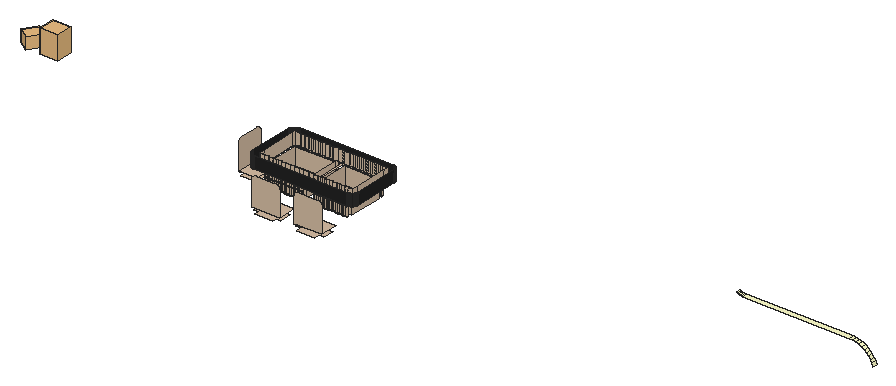
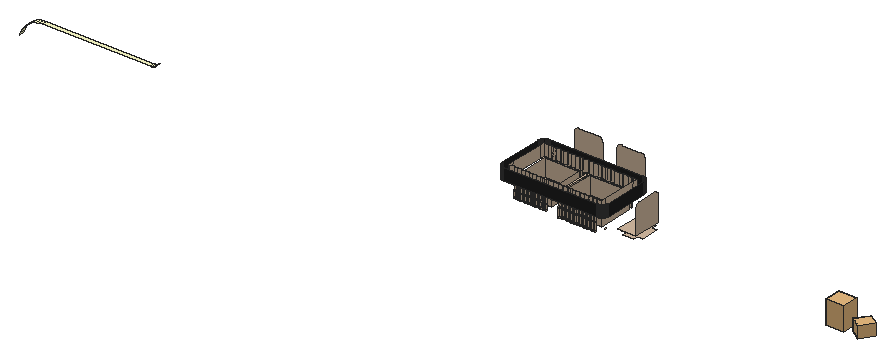
# SketchUp Ruby script. Lengths in inches.
U = 1.inch
M = Sketchup.active_model
def pt(a) = Geom::Point3d.new(a.map { |v| v * U })
def face(e, loops, mat)
  f = e.add_face(loops[0].map { |a| pt(a) })
  loops[1..].each { |l| e.add_face(l.map { |a| pt(a) }).erase! }
  f.material = f.back_material = mat if mat
  f
end
# faces: each face lists its corners as indices into pts; further lists are holes
def faces(e, pts, list, mat = nil) = list.each { |f| face(e, (f[0].is_a?(Array) ? f : [f]).map { |l| l.map { |i| pts[i] } }, mat) }
# xy, xz, yz: faces in a plane at the given z, y or x. An outline is a flat list of corners, or four numbers for a rectangle; further outlines are holes
def ring(l) = l.size == 4 ? [[l[0], l[1]], [l[2], l[1]], [l[2], l[3]], [l[0], l[3]]] : l.each_slice(2).to_a
def flat(e, list, mat, &to3) = list.each { |f| face(e, (f[0].is_a?(Array) ? f : [f]).map { |l| ring(l).map { |u, v| to3.(u, v) } }, mat) }
def xy(e, z, list, mat = nil) = flat(e, list, mat) { |x, y| [x, y, z] }
def xz(e, y, list, mat = nil) = flat(e, list, mat) { |x, z| [x, y, z] }
def yz(e, x, list, mat = nil) = flat(e, list, mat) { |y, z| [x, y, z] }
def lines(e, pts, list) = list.each { |a, b| e.add_line(pt(pts[a]), pt(pts[b])) }
# prism: a flat outline (further loops are holes) pulled along v
def prism(e, loops, v, mat = nil)
  f = face(e, loops, mat); d = Geom::Vector3d.new(v.map { |x| x * U })
  f.pushpull(f.normal.samedirection?(d) ? d.length : -d.length)
end
def box(e, o, s, mat = nil) = prism(e, [[o, [o[0] + s[0], o[1], o[2]], [o[0] + s[0], o[1] + s[1], o[2]], [o[0], o[1] + s[1], o[2]]]], [0, 0, s[2]], mat)
def at(x, y, z, deg = 0) = Geom::Transformation.translation(pt([x, y, z])) * Geom::Transformation.rotation(ORIGIN, Z_AXIS, deg.degrees)
def axes(o, x, y, z) = Geom::Transformation.new([*x, 0, *y, 0, *z, 0, *pt(o).to_a, 1])
def part(name) = M.definitions.add(name)
# library, detail: a bought-in or finely detailed component or shape, given as its bounding box
def library(name, o, s) = part(name).tap { |d| box(d.entities, o, s) }
def detail(e, o, s) = box(e.add_group.entities, o, s)
def put(e, d, t, mat = nil) = e.add_instance(d, t).tap { |i| i.material = mat if mat }
def group(e, t, mat = nil) = e.add_group.tap { |g| g.transformation = t; g.material = mat if mat }.entities
root = M.entities
M.materials.add("[0136_Charcoal]").color = [35, 35, 35]
M.materials.add("[Color E01]").color = [255, 255, 204]
M.materials.add("[Formica Laminate Light]").color = [213, 189, 164]
c1 = library("Vase 004",[-7.23,-6.39,-0.02],[13.74,12.68,17.81])
c2 = library("Books 155 025",[-5.0625,-5.83,0.01],[10.11,11.66,8.59])
xy(root,25.5625,[[268.91,97.95,268.91,101.59,265.27,101.59,265.27,110.07,268.72,110.07,268.72,113.72,282.83,113.72,282.83,110.07,286.47,110.07,286.47,101.59,282.83,101.59,282.83,97.95],[301.53,97.95,301.53,101.59,297.89,101.59,297.89,110.07,301.35,110.07,301.35,113.72,315.45,113.72,315.45,110.07,319.1,110.07,319.1,101.59,315.45,101.59,315.45,97.95],[233.08,129.3,233.08,132.94,229.44,132.94,229.44,146.86,233.08,146.86,233.08,150.5,241.57,150.5,241.57,147.05,245.21,147.05,245.21,132.94,241.57,132.94,241.57,129.3]],"[Formica Laminate Light]")
xy(root,26.83,[[255.19,159.08,257.64,160.01],[258.46,159.08,260.91,160.01],[261.72,159.08,264.17,160.01],[264.98,159.08,267.43,160.01],[268.24,159.08,270.69,160.01],
  [271.5,159.08,273.95,160.01],[274.76,159.08,277.21,160.01],[278.02,159.08,280.47,160.01],[281.29,159.08,283.74,160.01]],"[Formica Laminate Light]")
xy(root,27.63,[[255.19,159.08,257.64,160.01],[258.46,159.08,260.91,160.01],[261.72,159.08,264.17,160.01],[268.24,159.08,270.69,160.01],[271.5,159.08,273.95,160.01],
  [274.76,159.08,277.21,160.01],[278.02,159.08,280.47,160.01],[281.29,159.08,283.74,160.01]],"[Formica Laminate Light]")
xy(root,27.64,[[264.98,159.08,267.43,160.01]],"[Formica Laminate Light]")
xy(root,27.9,[[293.16,159.08,295.2,159.77],[296.03,159.08,298.0625,159.77],[298.89,159.08,300.93,159.77],[301.75,159.08,303.79,159.77],[304.62,159.08,306.66,159.77],
  [307.48,159.08,309.52,159.77],[310.35,159.08,312.38,159.77],[313.21,159.08,315.25,159.77],[316.07,159.08,318.11,159.77]],"[Formica Laminate Light]")
xy(root,28.25,[[265.27,99.82,286.47,113.72],[297.89,99.82,319.1,113.72],[231.32,129.3,245.21,150.5]],"[Formica Laminate Light]")
xy(root,28.4,[[254.81,124.84,257.68,125.33],[258.11,124.84,260.98,125.33],[261.41,124.84,264.28,125.33],[264.71,124.84,267.58,125.33],[268.02,124.84,270.89,125.33],
  [271.32,124.84,274.19,125.33],[274.625,124.84,277.49,125.33],[277.93,124.84,280.8,125.33],[281.23,124.84,284.1,125.33]],"[Formica Laminate Light]")
xy(root,28.69,[[254.38,128.96,284.55,155.08],[292.34,128.96,318.9375,155.08],[250.94,155.08,250.9,155.58,250.93,156.07,250.94,156.11],[293.16,159.08,295.2,159.77],[296.03,159.08,298.0625,159.77],
  [298.89,159.08,300.93,159.77],[301.75,159.08,303.79,159.77],[304.62,159.08,306.66,159.77],[307.48,159.08,309.52,159.77],[310.35,159.08,312.38,159.77],
  [313.21,159.08,315.25,159.77],[316.07,159.08,318.11,159.77]],"[Formica Laminate Light]")
xy(root,28.96,[[292.63,124.79,295.1875,125.33],[295.55,124.79,298.11,125.33],[298.47,124.79,301.04,125.33],[301.4,124.79,303.96,125.33],[304.32,124.79,306.88,125.33],
  [307.24,124.79,309.81,125.33],[310.17,124.79,312.73,125.33],[313.09,124.79,315.65,125.33],[316.01,124.79,318.58,125.33]],"[Formica Laminate Light]")
xy(root,32.6875,[[293.16,159.08,295.2,159.77],[296.03,159.08,298.0625,159.77],[298.89,159.08,300.93,159.77],[301.75,159.08,303.79,159.77],[304.62,159.08,306.66,159.77],
  [307.48,159.08,309.52,159.77],[310.35,159.08,312.38,159.77],[313.21,159.08,315.25,159.77],[316.07,159.08,318.11,159.77]],"[Formica Laminate Light]")
xy(root,33.4,[[255.19,159.08,257.64,160.01],[258.46,159.08,260.91,160.01],[261.72,159.08,264.17,160.01],[264.98,159.08,267.43,160.01],[268.24,159.08,270.69,160.01],
  [271.5,159.08,273.95,160.01],[274.76,159.08,277.21,160.01],[278.02,159.08,280.47,160.01],[281.29,159.08,283.74,160.01]],"[Formica Laminate Light]")
xy(root,33.49,[[293.16,159.08,295.2,159.77],[296.03,159.08,298.0625,159.77],[298.89,159.08,300.93,159.77],[301.75,159.08,303.79,159.77],[304.62,159.08,306.66,159.77],
  [307.48,159.08,309.52,159.77],[310.35,159.08,312.38,159.77],[313.21,159.08,315.25,159.77],[316.07,159.08,318.11,159.77]],"[Formica Laminate Light]")
xy(root,34.17,[[254.81,124.84,257.68,125.33],[258.11,124.84,260.98,125.33],[261.41,124.84,264.28,125.33],[264.71,124.84,267.58,125.33],[268.02,124.84,270.89,125.33],
  [271.32,124.84,274.19,125.33],[274.625,124.84,277.49,125.33],[277.93,124.84,280.8,125.33],[281.23,124.84,284.1,125.33]],"[Formica Laminate Light]")
xy(root,34.2,[[255.19,159.08,257.64,160.01],[258.46,159.08,260.91,160.01],[268.24,159.08,270.69,160.01],[271.5,159.08,273.95,160.01],[274.76,159.08,277.21,160.01],
  [278.02,159.08,280.47,160.01],[281.29,159.08,283.74,160.01]],"[Formica Laminate Light]")
xy(root,34.21,[[261.72,159.08,264.17,160.01]],"[Formica Laminate Light]")
xy(root,34.22,[[264.98,159.08,267.43,160.01]],"[Formica Laminate Light]")
xy(root,36.25,[[292.63,124.91,295.1875,125.45],[295.55,124.91,298.11,125.45],[298.47,124.91,301.04,125.45],[301.4,124.91,303.96,125.45],[304.32,124.91,306.88,125.45],
  [307.24,124.91,309.81,125.45],[310.17,124.91,312.73,125.45],[313.09,124.91,315.65,125.45],[316.01,124.91,318.58,125.45]],"[Formica Laminate Light]")
xy(root,39.6875,[[577,182.5625,659.67,185.9375]],"[Color E01]")
xy(root,40.33,[[[251.07,119.96,250.37,120,249.68,120.14,249.01,120.37,248.38,120.68,247.8,121.07,247.27,121.53,246.81,122.06,246.42,122.64,246.11,123.27,245.88,123.9375,245.74,124.625,245.7,125.33,245.7,159.08,245.8,159.73,245.97,160.35,246.22,160.95,246.54,161.52,246.93,162.04,247.39,162.51,247.89,162.91,248.44,163.26,249.03,163.53,249.65,163.73,250.29,163.85,250.94,163.89,322.35,163.89,323,163.85,323.63,163.73,324.24,163.53,324.82,163.25,325.37,162.91,325.86,162.5,326.3,162.03,326.68,161.51,326.99,160.94,327.22,160.34,327.38,159.72,327.46,159.08,327.46,125.33,327.42,124.65,327.29,123.98,327.08,123.33,326.78,122.72,326.42,122.14,325.98,121.62,325.48,121.16,324.93,120.76,324.33,120.44,323.69,120.2,323.03,120.03,322.35,119.96],[318.58,124.79,318.9375,124.79,318.9375,125.33,322.35,125.33,322.35,159.08,318.9375,159.08,318.9375,159.77,318.11,159.77,318.11,159.08,284.55,159.08,284.55,160.01,283.74,160.01,283.74,159.08,250.94,159.08,250.94,125.33,284.1,125.33,284.1,124.84,284.53,124.84,284.53,125.33,318.58,125.33]],[250.94,125.33,250.94,128.96,251.03,128.53,251.16,128.11,251.34,127.7,251.55,127.3125,251.81,126.95,252.09,126.61,252.42,126.3,252.77,126.03,253.14,125.79,253.54,125.6,253.95,125.44,254.38,125.33],[284.53,125.33,284.96,125.41,285.38,125.55,285.78,125.73,286.16,125.96,286.5,126.23,286.8125,126.55,287.08,126.89,287.31,127.27,287.49,127.67,287.62,128.09,287.69,128.53,287.72,128.96,287.72,125.33],[287.72,125.33,288.6,159.08],[288.6,125.33,288.6,129.05,288.63,128.5625,288.73,128.08,288.88,127.62,289.1,127.1875,289.37,126.78,289.6875,126.42,290.05,126.1,290.46,125.83,290.9,125.61,291.36,125.45,291.83,125.36,292.32,125.33],
  [318.9375,125.33,319.39,125.38,319.84,125.5,320.26,125.67,320.66,125.89,321.03,126.16,321.37,126.47,321.66,126.82,321.9,127.21,322.1,127.62,322.24,128.06,322.33,128.51,322.35,128.96,322.35,125.33],[287.72,155.08,287.7,155.54,287.62,155.99,287.49,156.43,287.32,156.86,287.1,157.26,286.83,157.63,286.53,157.98,286.1875,158.28,285.8125,158.55,285.41,158.77,284.99,158.95,284.55,159.08,287.72,159.08],[288.6,155.08,288.6,159.08,292.34,159.08,291.84,159.02,291.35,158.89,290.89,158.7,290.45,158.46,290.04,158.16,289.68,157.82,289.36,157.43,289.09,157.01,288.88,156.55,288.72,156.07,288.63,155.58],[322.35,155.08,322.33,155.56,322.24,156.03,322.1,156.48,321.91,156.92,321.67,157.33,321.38,157.71,321.05,158.05,320.69,158.36,320.28,158.62,319.85,158.82,319.4,158.98,318.9375,159.08,322.35,159.08],[250.94,156.11,250.94,159.08,254.38,159.08,253.88,159.05,253.4,158.94,252.93,158.76,252.49,158.52,252.09,158.22,251.74,157.87,251.45,157.47,251.21,157.03,251.04,156.5625]],"[Formica Laminate Light]")
xz(root,99.82,[[265.27,28.25,265.27,46.75,265.3,47.23,265.39,47.7,265.55,48.16,265.76,48.59,266.03,48.99,266.35,49.36,266.71,49.68,267.11,49.94,267.54,50.16,268,50.3125,268.47,50.41,268.95,50.4375,282.66,50.4375,283.14,50.41,283.61,50.32,284.0625,50.17,284.5,49.97,284.9,49.71,285.27,49.4,285.6,49.05,285.88,48.67,286.11,48.25,286.29,47.8,286.41,47.34,286.47,46.86,286.47,28.25],[297.89,28.25,297.89,46.82,297.92,47.26,298,47.69,298.13,48.12,298.3125,48.52,298.54,48.89,298.8125,49.24,299.125,49.55,299.47,49.82,299.85,50.05,300.26,50.23,300.68,50.36,301.11,50.4375,315.66,50.4375,316.125,50.41,316.58,50.3125,317.02,50.16,317.43,49.95,317.8125,49.68,318.15,49.37,318.45,49.01,318.7,48.61,318.89,48.1875,319.02,47.74,319.09,47.28,319.1,46.82,319.1,28.25]],"[Formica Laminate Light]")
xz(root,119.96,[[251.07,40.33,322.35,49.31]],"[0136_Charcoal]")
xz(root,124.79,[[292.63,28.96,295.1875,29.49],[295.55,28.96,298.11,29.49],[298.47,28.96,301.04,29.49],[301.4,28.96,303.96,29.49],[304.32,28.96,306.88,29.49],
  [307.24,28.96,309.81,29.49],[310.17,28.96,312.73,29.49],[313.09,28.96,315.65,29.49],[316.01,28.96,318.58,29.49]],"[Formica Laminate Light]")
xz(root,124.84,[[254.81,28.4,257.68,28.93],[258.11,28.4,260.98,28.93],[261.41,28.4,264.28,28.93],[264.71,28.4,267.58,28.93],[268.02,28.4,270.89,28.93],
  [271.32,28.4,274.19,28.93],[274.625,28.4,277.49,28.93],[277.93,28.4,280.8,28.93],[281.23,28.4,284.1,28.93],[254.81,34.17,257.68,34.71],
  [258.11,34.17,260.98,34.71],[261.41,34.17,264.28,34.71],[264.71,34.17,267.58,34.71],[268.02,34.17,270.89,34.71],[271.32,34.17,274.19,34.71],
  [274.625,34.17,277.49,34.71],[277.93,34.17,280.8,34.71],[281.23,34.17,284.1,34.71]],"[Formica Laminate Light]")
xz(root,124.91,[[292.63,36.25,295.1875,36.79],[295.55,36.25,298.11,36.79],[298.47,36.25,301.04,36.79],[301.4,36.25,303.96,36.79],[304.32,36.25,306.88,36.79],
  [307.24,36.25,309.81,36.79],[310.17,36.25,312.73,36.79],[313.09,36.25,315.65,36.79],[316.01,36.25,318.58,36.79]],"[Formica Laminate Light]")
xz(root,125.33,[[254.81,28.4,257.68,34.17],[258.11,28.4,260.98,34.17],[261.41,28.4,264.28,34.17],[264.71,28.4,267.58,34.17],[268.02,28.4,270.89,34.17],
  [271.32,28.4,274.19,34.17],[274.625,28.4,277.49,34.17],[277.93,28.4,280.8,34.17],[281.23,28.4,284.1,34.17],[292.63,28.96,295.1875,40.33],
  [295.55,28.96,298.11,40.33],[298.47,28.96,301.04,40.33],[301.4,28.96,303.96,40.33],[304.32,28.96,306.88,40.33],[307.24,28.96,309.81,40.33],
  [310.17,28.96,312.73,40.33],[313.09,28.96,315.65,40.33],[316.01,28.96,318.58,40.33],[254.81,34.17,257.68,40.33],[258.11,34.17,260.98,40.33],
  [261.41,34.17,264.28,40.33],[264.71,34.17,267.58,40.33],[268.02,34.17,270.89,40.33],[271.32,34.17,274.19,40.33],[274.625,34.17,277.49,40.33],
  [277.93,34.17,280.8,40.33],[281.23,34.17,284.1,40.33],[250.94,40.33,254.37,49.31],[254.37,40.33,254.38,49.31],[254.38,40.33,254.81,49.31],
  [254.81,40.33,257.68,49.31],[257.68,40.33,258.11,49.31],[258.11,40.33,260.98,49.31],[260.98,40.33,261.41,49.31],[261.41,40.33,264.28,49.31],
  [264.28,40.33,264.71,49.31],[264.71,40.33,267.58,49.31],[267.58,40.33,268.02,49.31],[268.02,40.33,270.89,49.31],[270.89,40.33,271.32,49.31],
  [271.32,40.33,274.19,49.31],[274.19,40.33,274.625,49.31],[274.625,40.33,277.49,49.31],[277.49,40.33,277.93,49.31],[277.93,40.33,280.8,49.31],
  [280.8,40.33,281.23,49.31],[281.23,40.33,284.1,49.31],[284.53,40.33,287.72,49.31],[287.72,40.33,288.6,49.31],[288.6,40.33,292.27,49.31],
  [292.27,40.33,292.32,49.31],[292.32,40.33,292.63,49.31],[292.63,40.33,295.1875,49.31],[295.1875,40.33,295.55,49.31],[295.55,40.33,298.11,49.31],
  [298.11,40.33,298.47,49.31],[298.47,40.33,301.04,49.31],[301.04,40.33,301.4,49.31],[301.4,40.33,303.96,49.31],[303.96,40.33,304.32,49.31],
  [304.32,40.33,306.88,49.31],[306.88,40.33,307.24,49.31],[307.24,40.33,309.81,49.31],[309.81,40.33,310.17,49.31],[310.17,40.33,312.73,49.31],
  [312.73,40.33,313.09,49.31],[313.09,40.33,315.65,49.31],[315.65,40.33,316.01,49.31],[316.01,40.33,318.58,49.31],[318.9375,40.33,322.35,49.31]],"[Formica Laminate Light]")
xz(root,128.96,[[254.38,28.69,284.55,41.75],[292.34,28.69,318.9375,41.67]],"[Formica Laminate Light]")
xz(root,155.08,[[254.38,28.69,284.55,41.75],[292.34,28.69,318.9375,41.67]],"[Formica Laminate Light]")
xz(root,159.08,[[255.19,26.83,257.64,27.63],[258.46,26.83,260.91,27.63],[261.72,26.83,264.17,27.63],[264.98,26.83,267.43,27.64],[268.24,26.83,270.69,27.63],
  [271.5,26.83,273.95,27.63],[274.76,26.83,277.21,27.63],[278.02,26.83,280.47,27.63],[281.29,26.83,283.74,27.63],[255.19,27.63,257.64,33.4],
  [258.46,27.63,260.91,33.4],[261.72,27.63,264.17,33.4],[268.24,27.63,270.69,33.4],[271.5,27.63,273.95,33.4],[274.76,27.63,277.21,33.4],
  [278.02,27.63,280.47,33.4],[281.29,27.63,283.74,33.4],[264.98,27.64,267.43,33.4],[293.16,27.9,295.2,28.69],[296.03,27.9,298.0625,28.69],
  [298.89,27.9,300.93,28.69],[301.75,27.9,303.79,28.69],[304.62,27.9,306.66,28.69],[307.48,27.9,309.52,28.69],[310.35,27.9,312.38,28.69],
  [313.21,27.9,315.25,28.69],[316.07,27.9,318.11,28.69],[293.16,28.69,295.2,32.6875],[296.03,28.69,298.0625,32.6875],[298.89,28.69,300.93,32.6875],
  [301.75,28.69,303.79,32.6875],[304.62,28.69,306.66,32.6875],[307.48,28.69,309.52,32.6875],[310.35,28.69,312.38,32.6875],[313.21,28.69,315.25,32.6875],
  [316.07,28.69,318.11,32.6875],[293.16,32.6875,295.2,33.49],[296.03,32.6875,298.0625,33.49],[298.89,32.6875,300.93,33.49],[301.75,32.6875,303.79,33.49],
  [304.62,32.6875,306.66,33.49],[307.48,32.6875,309.52,33.49],[310.35,32.6875,312.38,33.49],[313.21,32.6875,315.25,33.49],[316.07,32.6875,318.11,33.49],
  [255.19,33.4,257.64,34.2],[258.46,33.4,260.91,34.2],[261.72,33.4,264.17,34.21],[264.98,33.4,267.43,34.22],[268.24,33.4,270.69,34.2],
  [271.5,33.4,273.95,34.2],[274.76,33.4,277.21,34.2],[278.02,33.4,280.47,34.2],[281.29,33.4,283.74,34.2],[293.16,33.49,295.2,40.33],
  [296.03,33.49,298.0625,40.33],[298.89,33.49,300.93,40.33],[301.75,33.49,303.79,40.33],[304.62,33.49,306.66,40.33],[307.48,33.49,309.52,40.33],
  [310.35,33.49,312.38,40.33],[313.21,33.49,315.25,40.33],[316.07,33.49,318.11,40.33],[255.19,34.2,257.64,40.33],[258.46,34.2,260.91,40.33],
  [268.24,34.2,270.69,40.33],[271.5,34.2,273.95,40.33],[274.76,34.2,277.21,40.33],[278.02,34.2,280.47,40.33],[281.29,34.2,283.74,40.33],
  [261.72,34.21,264.17,40.33],[264.98,34.22,267.43,40.33],[250.94,40.33,254.38,49.31],[254.38,40.33,255.19,49.31],[255.19,40.33,257.64,49.31],
  [257.64,40.33,258.46,49.31],[258.46,40.33,260.91,49.31],[260.91,40.33,261.72,49.31],[261.72,40.33,264.17,49.31],[264.17,40.33,264.98,49.31],
  [264.98,40.33,267.43,49.31],[267.43,40.33,268.24,49.31],[268.24,40.33,270.69,49.31],[270.69,40.33,271.5,49.31],[271.5,40.33,273.95,49.31],
  [273.95,40.33,274.76,49.31],[274.76,40.33,277.21,49.31],[277.21,40.33,278.02,49.31],[278.02,40.33,280.47,49.31],[280.47,40.33,281.29,49.31],
  [281.29,40.33,283.74,49.31],[284.55,40.33,287.72,49.31],[287.72,40.33,288.6,49.31],[288.6,40.33,292.34,49.31],[292.34,40.33,292.97,49.31],
  [292.97,40.33,293.16,49.31],[293.16,40.33,295.2,49.31],[295.2,40.33,296.03,49.31],[296.03,40.33,298.0625,49.31],[298.0625,40.33,298.89,49.31],
  [298.89,40.33,300.93,49.31],[300.93,40.33,301.75,49.31],[301.75,40.33,303.79,49.31],[303.79,40.33,304.62,49.31],[304.62,40.33,306.66,49.31],
  [306.66,40.33,307.48,49.31],[307.48,40.33,309.52,49.31],[309.52,40.33,310.35,49.31],[310.35,40.33,312.38,49.31],[312.38,40.33,313.21,49.31],
  [313.21,40.33,315.25,49.31],[315.25,40.33,316.07,49.31],[316.07,40.33,318.11,49.31],[318.9375,40.33,322.35,49.31]],"[Formica Laminate Light]")
xz(root,159.77,[[293.16,27.9,295.2,28.69],[296.03,27.9,298.0625,28.69],[298.89,27.9,300.93,28.69],[301.75,27.9,303.79,28.69],[304.62,27.9,306.66,28.69],
  [307.48,27.9,309.52,28.69],[310.35,27.9,312.38,28.69],[313.21,27.9,315.25,28.69],[316.07,27.9,318.11,28.69],[293.16,32.6875,295.2,33.49],
  [296.03,32.6875,298.0625,33.49],[298.89,32.6875,300.93,33.49],[301.75,32.6875,303.79,33.49],[304.62,32.6875,306.66,33.49],[307.48,32.6875,309.52,33.49],
  [310.35,32.6875,312.38,33.49],[313.21,32.6875,315.25,33.49],[316.07,32.6875,318.11,33.49]],"[Formica Laminate Light]")
xz(root,160.01,[[255.19,26.83,257.64,27.63],[258.46,26.83,260.91,27.63],[261.72,26.83,264.17,27.63],[264.98,26.83,267.43,27.64],[268.24,26.83,270.69,27.63],
  [271.5,26.83,273.95,27.63],[274.76,26.83,277.21,27.63],[278.02,26.83,280.47,27.63],[281.29,26.83,283.74,27.63],[255.19,33.4,257.64,34.2],
  [258.46,33.4,260.91,34.2],[261.72,33.4,264.17,34.21],[264.98,33.4,267.43,34.22],[268.24,33.4,270.69,34.2],[271.5,33.4,273.95,34.2],
  [274.76,33.4,277.21,34.2],[278.02,33.4,280.47,34.2],[281.29,33.4,283.74,34.2]],"[Formica Laminate Light]")
xz(root,163.89,[[250.94,40.33,322.35,49.31]],"[0136_Charcoal]")
yz(root,231.32,[[129.3,28.25,150.5,28.25,150.5,46.75,150.47,47.23,150.38,47.7,150.22,48.16,150.01,48.59,149.74,48.99,149.42,49.36,149.06,49.68,148.66,49.94,148.23,50.16,147.77,50.3125,147.3,50.41,146.82,50.4375,133.11,50.4375,132.63,50.41,132.16,50.32,131.7,50.17,131.27,49.97,130.87,49.71,130.5,49.4,130.17,49.05,129.89,48.67,129.65,48.25,129.48,47.8,129.36,47.34,129.3,46.86]],"[Formica Laminate Light]")
yz(root,245.7,[[125.33,40.33,159.08,49.31]],"[0136_Charcoal]")
yz(root,250.94,[[125.33,40.33,128.96,49.31],[128.96,40.33,156.11,49.31],[156.11,40.33,159.08,49.31]],"[Formica Laminate Light]")
yz(root,254.38,[[128.96,28.69,155.08,41.75]],"[Formica Laminate Light]")
yz(root,254.81,[[124.84,28.4,125.33,34.17],[124.84,34.17,125.33,40.33]],"[Formica Laminate Light]")
yz(root,255.19,[[159.08,26.83,160.01,27.63],[159.08,27.63,160.01,33.4],[159.08,33.4,160.01,34.2],[159.08,34.2,160.01,40.33]],"[Formica Laminate Light]")
yz(root,257.64,[[159.08,26.83,160.01,27.63],[159.08,27.63,160.01,33.4],[159.08,33.4,160.01,34.2],[159.08,34.2,160.01,40.33]],"[Formica Laminate Light]")
yz(root,257.68,[[124.84,28.4,125.33,34.17],[124.84,34.17,125.33,40.33]],"[Formica Laminate Light]")
yz(root,258.11,[[124.84,28.4,125.33,34.17],[124.84,34.17,125.33,40.33]],"[Formica Laminate Light]")
yz(root,258.46,[[159.08,26.83,160.01,27.63],[159.08,27.63,160.01,33.4],[159.08,33.4,160.01,34.2],[159.08,34.2,160.01,40.33]],"[Formica Laminate Light]")
yz(root,260.91,[[159.08,26.83,160.01,27.63],[159.08,27.63,160.01,33.4],[159.08,33.4,160.01,34.2],[159.08,34.2,160.01,40.33]],"[Formica Laminate Light]")
yz(root,260.98,[[124.84,28.4,125.33,34.17],[124.84,34.17,125.33,40.33]],"[Formica Laminate Light]")
yz(root,261.41,[[124.84,28.4,125.33,34.17],[124.84,34.17,125.33,40.33]],"[Formica Laminate Light]")
yz(root,261.72,[[159.08,26.83,160.01,27.63],[159.08,27.63,160.01,33.4],[159.08,33.4,160.01,34.21],[159.08,34.21,160.01,40.33]],"[Formica Laminate Light]")
yz(root,264.17,[[159.08,26.83,160.01,27.63],[159.08,27.63,160.01,33.4],[159.08,33.4,160.01,34.21],[159.08,34.21,160.01,40.33]],"[Formica Laminate Light]")
yz(root,264.28,[[124.84,28.4,125.33,34.17],[124.84,34.17,125.33,40.33]],"[Formica Laminate Light]")
yz(root,264.71,[[124.84,28.4,125.33,34.17],[124.84,34.17,125.33,40.33]],"[Formica Laminate Light]")
yz(root,264.98,[[159.08,26.83,160.01,27.64],[159.08,27.64,160.01,33.4],[159.08,33.4,160.01,34.22],[159.08,34.22,160.01,40.33]],"[Formica Laminate Light]")
yz(root,267.43,[[159.08,26.83,160.01,27.64],[159.08,27.64,160.01,33.4],[159.08,33.4,160.01,34.22],[159.08,34.22,160.01,40.33]],"[Formica Laminate Light]")
yz(root,267.58,[[124.84,28.4,125.33,34.17],[124.84,34.17,125.33,40.33]],"[Formica Laminate Light]")
yz(root,268.02,[[124.84,28.4,125.33,34.17],[124.84,34.17,125.33,40.33]],"[Formica Laminate Light]")
yz(root,268.24,[[159.08,26.83,160.01,27.63],[159.08,27.63,160.01,33.4],[159.08,33.4,160.01,34.2],[159.08,34.2,160.01,40.33]],"[Formica Laminate Light]")
yz(root,270.69,[[159.08,26.83,160.01,27.63],[159.08,27.63,160.01,33.4],[159.08,33.4,160.01,34.2],[159.08,34.2,160.01,40.33]],"[Formica Laminate Light]")
yz(root,270.89,[[124.84,28.4,125.33,34.17],[124.84,34.17,125.33,40.33]],"[Formica Laminate Light]")
yz(root,271.32,[[124.84,28.4,125.33,34.17],[124.84,34.17,125.33,40.33]],"[Formica Laminate Light]")
yz(root,271.5,[[159.08,26.83,160.01,27.63],[159.08,27.63,160.01,33.4],[159.08,33.4,160.01,34.2],[159.08,34.2,160.01,40.33]],"[Formica Laminate Light]")
yz(root,273.95,[[159.08,26.83,160.01,27.63],[159.08,27.63,160.01,33.4],[159.08,33.4,160.01,34.2],[159.08,34.2,160.01,40.33]],"[Formica Laminate Light]")
yz(root,274.19,[[124.84,28.4,125.33,34.17],[124.84,34.17,125.33,40.33]],"[Formica Laminate Light]")
yz(root,274.625,[[124.84,28.4,125.33,34.17],[124.84,34.17,125.33,40.33]],"[Formica Laminate Light]")
yz(root,274.76,[[159.08,26.83,160.01,27.63],[159.08,27.63,160.01,33.4],[159.08,33.4,160.01,34.2],[159.08,34.2,160.01,40.33]],"[Formica Laminate Light]")
yz(root,277.21,[[159.08,26.83,160.01,27.63],[159.08,27.63,160.01,33.4],[159.08,33.4,160.01,34.2],[159.08,34.2,160.01,40.33]],"[Formica Laminate Light]")
yz(root,277.49,[[124.84,28.4,125.33,34.17],[124.84,34.17,125.33,40.33]],"[Formica Laminate Light]")
yz(root,277.93,[[124.84,28.4,125.33,34.17],[124.84,34.17,125.33,40.33]],"[Formica Laminate Light]")
yz(root,278.02,[[159.08,26.83,160.01,27.63],[159.08,27.63,160.01,33.4],[159.08,33.4,160.01,34.2],[159.08,34.2,160.01,40.33]],"[Formica Laminate Light]")
yz(root,280.47,[[159.08,26.83,160.01,27.63],[159.08,27.63,160.01,33.4],[159.08,33.4,160.01,34.2],[159.08,34.2,160.01,40.33]],"[Formica Laminate Light]")
yz(root,280.8,[[124.84,28.4,125.33,34.17],[124.84,34.17,125.33,40.33]],"[Formica Laminate Light]")
yz(root,281.23,[[124.84,28.4,125.33,34.17],[124.84,34.17,125.33,40.33]],"[Formica Laminate Light]")
yz(root,281.29,[[159.08,26.83,160.01,27.63],[159.08,27.63,160.01,33.4],[159.08,33.4,160.01,34.2],[159.08,34.2,160.01,40.33]],"[Formica Laminate Light]")
yz(root,283.74,[[159.08,26.83,160.01,27.63],[159.08,27.63,160.01,33.4],[159.08,33.4,160.01,34.2]],"[Formica Laminate Light]")
yz(root,284.1,[[124.84,28.4,125.33,34.17]],"[Formica Laminate Light]")
yz(root,284.55,[[128.96,28.69,155.08,41.75]],"[Formica Laminate Light]")
yz(root,292.34,[[128.96,28.69,155.08,41.67]],"[Formica Laminate Light]")
yz(root,292.63,[[124.79,28.96,125.33,40.33]],"[Formica Laminate Light]")
yz(root,293.16,[[159.08,27.9,159.77,28.69],[159.08,28.69,159.77,32.6875],[159.08,32.6875,159.77,33.49],[159.08,33.49,159.77,40.33]],"[Formica Laminate Light]")
yz(root,295.1875,[[124.79,28.96,125.33,40.33]],"[Formica Laminate Light]")
yz(root,295.2,[[159.08,27.9,159.77,28.69],[159.08,28.69,159.77,32.6875],[159.08,32.6875,159.77,33.49],[159.08,33.49,159.77,40.33]],"[Formica Laminate Light]")
yz(root,295.55,[[124.79,28.96,125.33,40.33]],"[Formica Laminate Light]")
yz(root,296.03,[[159.08,27.9,159.77,28.69],[159.08,28.69,159.77,32.6875],[159.08,32.6875,159.77,33.49],[159.08,33.49,159.77,40.33]],"[Formica Laminate Light]")
yz(root,298.0625,[[159.08,27.9,159.77,28.69],[159.08,28.69,159.77,32.6875],[159.08,32.6875,159.77,33.49],[159.08,33.49,159.77,40.33]],"[Formica Laminate Light]")
yz(root,298.11,[[124.79,28.96,125.33,40.33]],"[Formica Laminate Light]")
yz(root,298.47,[[124.79,28.96,125.33,40.33]],"[Formica Laminate Light]")
yz(root,298.89,[[159.08,27.9,159.77,28.69],[159.08,28.69,159.77,32.6875],[159.08,32.6875,159.77,33.49],[159.08,33.49,159.77,40.33]],"[Formica Laminate Light]")
yz(root,300.93,[[159.08,27.9,159.77,28.69],[159.08,28.69,159.77,32.6875],[159.08,32.6875,159.77,33.49],[159.08,33.49,159.77,40.33]],"[Formica Laminate Light]")
yz(root,301.04,[[124.79,28.96,125.33,40.33]],"[Formica Laminate Light]")
yz(root,301.4,[[124.79,28.96,125.33,40.33]],"[Formica Laminate Light]")
yz(root,301.75,[[159.08,27.9,159.77,28.69],[159.08,28.69,159.77,32.6875],[159.08,32.6875,159.77,33.49],[159.08,33.49,159.77,40.33]],"[Formica Laminate Light]")
yz(root,303.79,[[159.08,27.9,159.77,28.69],[159.08,28.69,159.77,32.6875],[159.08,32.6875,159.77,33.49],[159.08,33.49,159.77,40.33]],"[Formica Laminate Light]")
yz(root,303.96,[[124.79,28.96,125.33,40.33]],"[Formica Laminate Light]")
yz(root,304.32,[[124.79,28.96,125.33,40.33]],"[Formica Laminate Light]")
yz(root,304.62,[[159.08,27.9,159.77,28.69],[159.08,28.69,159.77,32.6875],[159.08,32.6875,159.77,33.49],[159.08,33.49,159.77,40.33]],"[Formica Laminate Light]")
yz(root,306.66,[[159.08,27.9,159.77,28.69],[159.08,28.69,159.77,32.6875],[159.08,32.6875,159.77,33.49],[159.08,33.49,159.77,40.33]],"[Formica Laminate Light]")
yz(root,306.88,[[124.79,28.96,125.33,40.33]],"[Formica Laminate Light]")
yz(root,307.24,[[124.79,28.96,125.33,40.33]],"[Formica Laminate Light]")
yz(root,307.48,[[159.08,27.9,159.77,28.69],[159.08,28.69,159.77,32.6875],[159.08,32.6875,159.77,33.49],[159.08,33.49,159.77,40.33]],"[Formica Laminate Light]")
yz(root,309.52,[[159.08,27.9,159.77,28.69],[159.08,28.69,159.77,32.6875],[159.08,32.6875,159.77,33.49],[159.08,33.49,159.77,40.33]],"[Formica Laminate Light]")
yz(root,309.81,[[124.79,28.96,125.33,40.33]],"[Formica Laminate Light]")
yz(root,310.17,[[124.79,28.96,125.33,40.33]],"[Formica Laminate Light]")
yz(root,310.35,[[159.08,27.9,159.77,28.69],[159.08,28.69,159.77,32.6875],[159.08,32.6875,159.77,33.49],[159.08,33.49,159.77,40.33]],"[Formica Laminate Light]")
yz(root,312.38,[[159.08,27.9,159.77,28.69],[159.08,28.69,159.77,32.6875],[159.08,32.6875,159.77,33.49],[159.08,33.49,159.77,40.33]],"[Formica Laminate Light]")
yz(root,312.73,[[124.79,28.96,125.33,40.33]],"[Formica Laminate Light]")
yz(root,313.09,[[124.79,28.96,125.33,40.33]],"[Formica Laminate Light]")
yz(root,313.21,[[159.08,27.9,159.77,28.69],[159.08,28.69,159.77,32.6875],[159.08,32.6875,159.77,33.49],[159.08,33.49,159.77,40.33]],"[Formica Laminate Light]")
yz(root,315.25,[[159.08,27.9,159.77,28.69],[159.08,28.69,159.77,32.6875],[159.08,32.6875,159.77,33.49],[159.08,33.49,159.77,40.33]],"[Formica Laminate Light]")
yz(root,315.65,[[124.79,28.96,125.33,40.33]],"[Formica Laminate Light]")
yz(root,316.01,[[124.79,28.96,125.33,40.33]],"[Formica Laminate Light]")
yz(root,316.07,[[159.08,27.9,159.77,28.69],[159.08,28.69,159.77,32.6875],[159.08,32.6875,159.77,33.49],[159.08,33.49,159.77,40.33]],"[Formica Laminate Light]")
yz(root,318.11,[[159.08,27.9,159.77,28.69],[159.08,28.69,159.77,32.6875],[159.08,32.6875,159.77,33.49]],"[Formica Laminate Light]")
yz(root,318.9375,[[128.96,28.69,155.08,41.67]],"[Formica Laminate Light]")
yz(root,322.35,[[125.33,40.33,128.96,49.31],[128.96,40.33,155.08,49.31],[155.08,40.33,159.08,49.31]],"[Formica Laminate Light]")
yz(root,327.46,[[125.33,40.33,159.08,49.31]],"[0136_Charcoal]")
p = [[676.38,185.9375,28.52],[676.38,182.5625,28.52],[677.14,182.5625,26.28],[677.14,185.9375,26.28],[675.34,185.9375,30.64],[675.34,182.5625,30.64],
  [674.02,185.9375,32.61],[674.02,182.5625,32.61],[672.46,185.9375,34.39],[672.46,182.5625,34.39],[670.68,185.9375,35.95],[670.68,182.5625,35.95],
  [668.72,185.9375,37.26],[668.72,182.5625,37.26],[666.6,185.9375,38.3125],[666.6,182.5625,38.3125],[664.36,185.9375,39.07],[664.36,182.5625,39.07],
  [662.04,185.9375,39.53],[662.04,182.5625,39.53],[659.67,185.9375,39.6875],[659.67,182.5625,39.6875],[575.96,185.9375,39.76],[575.96,182.5625,39.76],
  [577,182.5625,39.6875],[577,185.9375,39.6875],[574.93,185.9375,39.96],[574.93,182.5625,39.96],[573.94,185.9375,40.3],[573.94,182.5625,40.3],
  [249.68,120.14,40.33],[250.37,120,40.33],[250.37,120,49.31],[249.68,120.14,49.31],[251.07,119.96,40.33],[251.07,119.96,49.31],
  [322.35,119.96,40.33],[323.03,120.03,40.33],[323.03,120.03,49.31],[322.35,119.96,49.31],[323.69,120.2,40.33],[323.69,120.2,49.31],
  [249.01,120.37,40.33],[249.01,120.37,49.31],[324.33,120.44,40.33],[324.33,120.44,49.31],[248.38,120.68,40.33],[248.38,120.68,49.31],
  [324.93,120.76,40.33],[324.93,120.76,49.31],[247.8,121.07,40.33],[247.8,121.07,49.31],[325.48,121.16,40.33],[325.48,121.16,49.31],
  [247.27,121.53,40.33],[247.27,121.53,49.31],[325.98,121.62,40.33],[325.98,121.62,49.31],[246.81,122.06,40.33],[246.81,122.06,49.31],
  [326.42,122.14,40.33],[326.42,122.14,49.31],[246.42,122.64,40.33],[246.42,122.64,49.31],[326.78,122.72,40.33],[326.78,122.72,49.31],
  [246.11,123.27,40.33],[246.11,123.27,49.31],[327.08,123.33,40.33],[327.08,123.33,49.31],[245.88,123.9375,40.33],[245.88,123.9375,49.31],
  [327.29,123.98,40.33],[327.29,123.98,49.31],[245.74,124.625,40.33],[245.74,124.625,49.31],[327.42,124.65,40.33],[327.42,124.65,49.31],
  [245.7,125.33,40.33],[245.7,125.33,49.31],[327.46,125.33,40.33],[327.46,125.33,49.31],[245.8,159.73,40.33],[245.7,159.08,40.33],
  [245.7,159.08,49.31],[245.8,159.73,49.31],[327.46,159.08,40.33],[327.38,159.72,40.33],[327.38,159.72,49.31],[327.46,159.08,49.31],
  [245.97,160.35,40.33],[245.97,160.35,49.31],[327.22,160.34,40.33],[327.22,160.34,49.31],[326.99,160.94,40.33],[326.99,160.94,49.31],
  [246.22,160.95,40.33],[246.22,160.95,49.31],[326.68,161.51,40.33],[326.68,161.51,49.31],[246.54,161.52,40.33],[246.54,161.52,49.31],
  [246.93,162.04,40.33],[246.93,162.04,49.31],[326.3,162.03,40.33],[326.3,162.03,49.31],[247.39,162.51,40.33],[247.39,162.51,49.31],
  [325.86,162.5,40.33],[325.86,162.5,49.31],[247.89,162.91,40.33],[247.89,162.91,49.31],[325.37,162.91,40.33],[325.37,162.91,49.31],
  [248.44,163.26,40.33],[248.44,163.26,49.31],[324.82,163.25,40.33],[324.82,163.25,49.31],[249.03,163.53,40.33],[249.03,163.53,49.31],
  [324.24,163.53,40.33],[324.24,163.53,49.31],[249.65,163.73,40.33],[249.65,163.73,49.31],[323.63,163.73,40.33],[323.63,163.73,49.31],
  [250.29,163.85,40.33],[250.29,163.85,49.31],[323,163.85,40.33],[323,163.85,49.31],[250.94,163.89,40.33],[250.94,163.89,49.31],
  [322.35,163.89,40.33],[322.35,163.89,49.31],[573.01,185.9375,40.76],[573.01,182.5625,40.76],[572.14,185.9375,41.34],[572.14,182.5625,41.34],
  [318.58,124.79,40.33],[318.58,124.79,29.49],[284.1,124.84,40.33],[284.1,124.84,34.71],[318.11,159.77,40.33],[318.11,159.77,33.49],
  [283.74,160.01,40.33],[283.74,160.01,34.2],[284.1,124.84,49.31],[284.53,124.84,40.33],[284.53,124.84,49.31],[318.58,124.79,49.31],
  [318.9375,124.79,40.33],[318.9375,124.79,49.31],[318.9375,159.77,40.33],[318.9375,159.77,49.31],[318.11,159.77,49.31],[284.55,160.01,40.33],
  [284.55,160.01,49.31],[283.74,160.01,49.31]]
faces(root,p,[[0,1,2,3],[4,5,1,0],[6,7,5,4],[8,9,7,6],[10,11,9,8],[12,13,11,10],[14,15,13,12],[16,17,15,14],
  [18,19,17,16],[20,21,19,18],[22,23,24,25],[26,27,23,22],[28,29,27,26],[134,135,29,28],[136,137,135,134]],"[Color E01]")
faces(root,p,[[30,31,32,33],[31,34,35,32],[36,37,38,39],[37,40,41,38],[42,30,33,43],[40,44,45,41],[46,42,43,47],[44,48,49,45],
  [50,46,47,51],[48,52,53,49],[54,50,51,55],[52,56,57,53],[58,54,55,59],[56,60,61,57],[62,58,59,63],[60,64,65,61],
  [66,62,63,67],[64,68,69,65],[70,66,67,71],[68,72,73,69],[74,70,71,75],[72,76,77,73],[78,74,75,79],[76,80,81,77],
  [82,83,84,85],[86,87,88,89],[90,82,85,91],[87,92,93,88],[92,94,95,93],[96,90,91,97],[94,98,99,95],[100,96,97,101],
  [102,100,101,103],[98,104,105,99],[106,102,103,107],[104,108,109,105],[110,106,107,111],[108,112,113,109],[114,110,111,115],[112,116,117,113],
  [118,114,115,119],[116,120,121,117],[122,118,119,123],[120,124,125,121],[126,122,123,127],[124,128,129,125],[130,126,127,131],[128,132,133,129]],"[0136_Charcoal]")
lines(root,p,[[138,139],[140,141],[142,143],[144,145],[140,146],[147,148],[138,149],[150,151],[152,153],[142,154],[155,156],[144,157]])
put(root,c1,at(61.75,165.64,33.77),"[Formica Laminate Light]")
put(root,c2,at(43.48,165.49,33.77,-33.9),"[Formica Laminate Light]")
